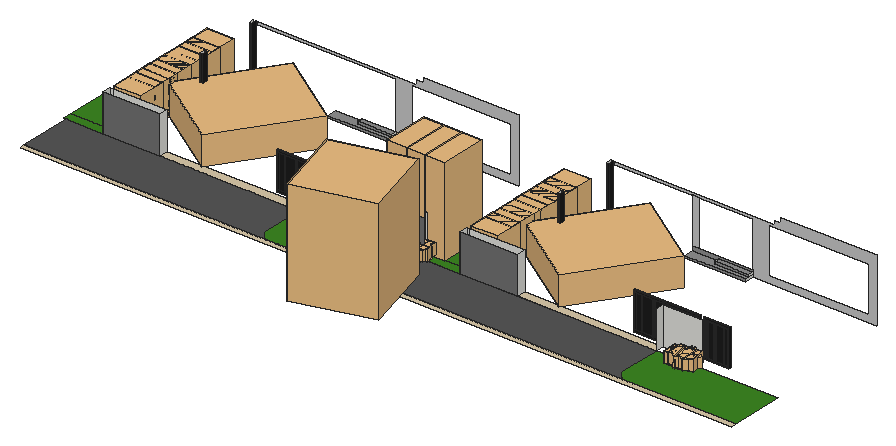
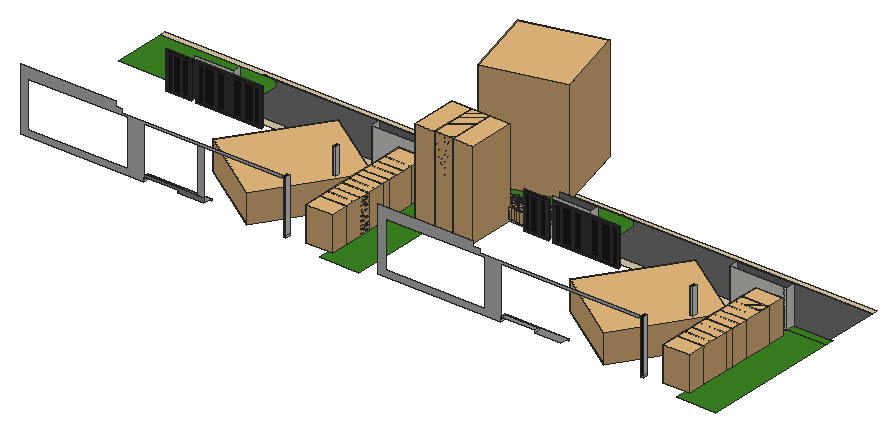
# SketchUp Ruby script. Lengths in inches.
U = 1.inch
M = Sketchup.active_model
def pt(a) = Geom::Point3d.new(a.map { |v| v * U })
def face(e, loops, mat)
  f = e.add_face(loops[0].map { |a| pt(a) })
  loops[1..].each { |l| e.add_face(l.map { |a| pt(a) }).erase! }
  f.material = f.back_material = mat if mat
  f
end
# faces: each face lists its corners as indices into pts; further lists are holes
def faces(e, pts, list, mat = nil) = list.each { |f| face(e, (f[0].is_a?(Array) ? f : [f]).map { |l| l.map { |i| pts[i] } }, mat) }
# xy, xz, yz: faces in a plane at the given z, y or x. An outline is a flat list of corners, or four numbers for a rectangle; further outlines are holes
def ring(l) = l.size == 4 ? [[l[0], l[1]], [l[2], l[1]], [l[2], l[3]], [l[0], l[3]]] : l.each_slice(2).to_a
def flat(e, list, mat, &to3) = list.each { |f| face(e, (f[0].is_a?(Array) ? f : [f]).map { |l| ring(l).map { |u, v| to3.(u, v) } }, mat) }
def xy(e, z, list, mat = nil) = flat(e, list, mat) { |x, y| [x, y, z] }
def xz(e, y, list, mat = nil) = flat(e, list, mat) { |x, z| [x, y, z] }
def yz(e, x, list, mat = nil) = flat(e, list, mat) { |y, z| [x, y, z] }
def lines(e, pts, list) = list.each { |a, b| e.add_line(pt(pts[a]), pt(pts[b])) }
# prism: a flat outline (further loops are holes) pulled along v
def prism(e, loops, v, mat = nil)
  f = face(e, loops, mat); d = Geom::Vector3d.new(v.map { |x| x * U })
  f.pushpull(f.normal.samedirection?(d) ? d.length : -d.length)
end
def box(e, o, s, mat = nil) = prism(e, [[o, [o[0] + s[0], o[1], o[2]], [o[0] + s[0], o[1] + s[1], o[2]], [o[0], o[1] + s[1], o[2]]]], [0, 0, s[2]], mat)
def at(x, y, z, deg = 0) = Geom::Transformation.translation(pt([x, y, z])) * Geom::Transformation.rotation(ORIGIN, Z_AXIS, deg.degrees)
def axes(o, x, y, z) = Geom::Transformation.new([*x, 0, *y, 0, *z, 0, *pt(o).to_a, 1])
def part(name) = M.definitions.add(name)
# library, detail: a bought-in or finely detailed component or shape, given as its bounding box
def library(name, o, s) = part(name).tap { |d| box(d.entities, o, s) }
def detail(e, o, s) = box(e.add_group.entities, o, s)
def put(e, d, t, mat = nil) = e.add_instance(d, t).tap { |i| i.material = mat if mat }
def group(e, t, mat = nil) = e.add_group.tap { |g| g.transformation = t; g.material = mat if mat }.entities
root = M.entities
M.materials.add("[Color M02]").color = [198, 198, 198]
M.materials.add("[Color M04]").color = [60, 133, 34]
M.materials.add("[Color M04]1").color = [142, 142, 142]
M.materials.add("[Color M05]1").color = [114, 114, 114]
M.materials.add("[Color M08]").color = [30, 30, 30]
M.materials.add("[Color_F16]").color = [51, 102, 0]
M.materials.add("[Field Square Tile]").color = [217, 201, 169]
M.materials.add("[Slate Light Tile]").color = [86, 86, 86]
c1 = library("plant (1)",[-35.72,-28.42,0],[66.31,67.39,84.38])
c2 = library("002+Bmw+M4+++mat3.4+2017",[-252.8,19.48,9.01],[196.94,171.32,55.15])
c3 = part("Group\#102")
g1 = group(c3.entities,at(0,0,0))
prism(g1,[[[0,3,72],[70.5,3,72],[70.5,3,0],[0,3,0]],[[67.5,3,3],[67.5,3,69],[3,3,69],[3,3,3]]],[0,-3,0])
c4 = part("Group\#135")
box(c4.entities,[0,0,0],[0.5,1,66])
c5 = part("Group\#148")
box(c5.entities,[0,-1,0],[5.5,1,66])
box(c5.entities,[50.84,-1,0],[13.66,1,66])
box(c5.entities,[28.06,-1,0],[22.28,1,66])
box(c5.entities,[24.66,-1,0],[2.9,1,66])
box(c5.entities,[6,-1,0],[18.16,1,66])
c6 = part("Component\#23")
g2 = group(c6.entities,at(70.5,0,0),"[Color M08]")
put(g2,c3,axes([70.5,0,0],[-1,0,0],[0,1,0],[0,0,1]))
g3 = group(g2,at(3,2,3))
g4 = group(g3,at(0,-1,0))
box(g4,[0,0,0],[5.5,1,66])
box(g4,[50.84,0,0],[13.66,1,66])
box(g4,[28.06,0,0],[22.28,1,66])
box(g4,[24.66,0,0],[2.9,1,66])
box(g4,[6,0,0],[18.16,1,66])
put(g3,c4,axes([50.34,0,0],[1,0,0],[0,-1,0],[0,0,1]))
put(g3,c4,axes([24.16,0,0],[1,0,0],[0,-1,0],[0,0,1]))
put(g3,c4,axes([27.56,0,0],[1,0,0],[0,-1,0],[0,0,1]))
put(g3,c4,axes([5.5,0,0],[1,0,0],[0,-1,0],[0,0,1]))
g5 = group(c6.entities,at(70.5,0,0),"[Color M08]")
put(g5,c3,at(-70.5,0,0))
g6 = group(g5,at(-3,2,3,-180))
put(g6,c5,at(0,1,0))
put(g6,c4,at(50.34,0,0))
put(g6,c4,at(24.16,0,0))
put(g6,c4,at(27.56,0,0))
put(g6,c4,at(5.5,0,0))
g7 = group(c6.entities,at(150,0,0),"[Color M08]")
put(g7,c3,axes([54,0,0],[-0.76596,0,0],[0,1,0],[0,0,1]))
g8 = group(g7,at(2.3,2,3))
put(g8,c5,axes([0,-1,0],[0.76596,0,0],[0,-1,0],[0,0,1]))
put(g8,c4,axes([38.55,0,0],[0.76596,0,0],[0,-1,0],[0,0,1]))
put(g8,c4,axes([18.5,0,0],[0.76596,0,0],[0,-1,0],[0,0,1]))
put(g8,c4,axes([21.11,0,0],[0.76596,0,0],[0,-1,0],[0,0,1]))
put(g8,c4,axes([4.22,0,0],[0.76596,0,0],[0,-1,0],[0,0,1]))
c7 = library("Obj_000004",[-25.54,-25.36,-14.31],[50.67,50.64,41.42])
c8 = library("Obj_000003",[-31,-31.06,-7.89],[62,62.12,39.58])
c9 = library("Potted plant",[-29.7,0,-10.87],[31.67,38.52,72.45])
c10 = library("Palm tree",[-4.09,-4.52,0],[193.52,193.51,258.93])
c11 = part("Palm+Tree")
put(c11.entities,c10,at(25.51,-21.81,0,15))
xy(root,-19.75,[[690.23,10.6,695.34,11.14,700.32,12.39,677.89,12.39,680.03,11.68,685.09,10.78],[1576.69,10.6,1581.8,11.14,1586.78,12.39,1564.35,12.39,1566.5,11.68,1571.56,10.78],[749.87,12.09,755.08,12.39,743.38,12.39,744.65,12.24],[165.7,143.39,173.14,164.82],[173.14,143.39,308.39,164.82],
  [1052.17,143.39,1059.6,164.82],[1059.6,143.39,1194.85,164.82],[264.14,322.71,270.875,334.4375],[1150.61,322.71,1157.34,334.4375],[264.14,475.3125,270.875,487.3125],
  [1150.61,475.3125,1157.34,487.3125]])
xy(root,-19.75,[[677.89,12.39,955.37,12.39,955.37,143.39,653.09,143.39,653.09,39.89,654.46,34.93,656.52,30.23,659.21,25.85,662.49,21.9,666.29,18.4375,670.54,15.55,675.15,13.28],[955.37,12.39,962.46,143.39],[1564.35,12.39,1841.83,12.39,1841.83,143.39,1539.55,143.39,1539.55,39.89,1540.93,34.93,1542.98,30.23,1545.68,25.85,1548.96,21.9,1552.76,18.4375,1557.01,15.55,1561.62,13.28],[68.91,143.39,165.7,164.82],[955.37,143.39,1052.17,164.82],
  [68.91,164.82,165.7,505.3125],[955.37,164.82,1052.17,505.3125]],"[Color M04]")
xy(root,-19.75,[[308.39,143.39,653.09,164.82],[1194.85,143.39,1539.55,164.82]],"[Field Square Tile]")
xy(root,-19.75,[[75.99,12.39,677.89,12.39,675.15,13.28,670.54,15.55,666.29,18.4375,662.49,21.9,659.21,25.85,656.52,30.23,654.46,34.93,653.09,39.89,653.09,143.39,75.99,143.39],[962.46,12.39,1564.35,12.39,1561.62,13.28,1557.01,15.55,1552.76,18.4375,1548.96,21.9,1545.68,25.85,1542.98,30.23,1540.93,34.93,1539.55,39.89,1539.55,143.39,962.46,143.39]],"[Slate Light Tile]")
xy(root,-19.3125,[[75.99,0,955.37,12.39],[955.37,0,962.46,12.39],[962.46,0,1841.83,12.39]],"[Field Square Tile]")
xy(root,-14.01,[[468.02,464.0625,618.43,464.0625,618.43,474.5625,534.06,474.5625,534.06,487.3125,468.02,487.3125],[1354.48,464.0625,1504.89,464.0625,1504.89,474.5625,1420.52,474.5625,1420.52,487.3125,1354.48,487.3125]],"[Color M04]1")
xy(root,-8.01,[[534.06,474.5625,618.43,487.3125],[1420.52,474.5625,1504.89,487.3125]],"[Color M04]1")
xz(root,12.39,[[75.99,-19.75,700.32,-19.3125],[700.32,-19.75,955.37,-19.3125],[955.37,-19.75,962.46,-19.3125],[962.46,-19.75,1586.78,-19.3125]])
xz(root,143.39,[[165.7,-19.75,308.39,73],[653.09,-19.75,962.46,-19.75,962.46,73,901.18,73,901.18,9.9375,747.55,9.9375,747.55,73,653.09,73],[1052.17,-19.75,1194.85,73]],"[Color M05]1")
xz(root,164.82,[[165.7,-19.75,173.14,73],[173.14,-19.75,173.14,73,308.39,73,308.39,-19.75,274.58,-19.75,274.58,-15.625,260.77,-15.625,260.77,-19.75],[260.77,-19.75,274.58,-15.625],[653.09,-19.75,747.55,73],[747.55,-19.75,901.18,9.9375],
  [901.18,-19.75,951.9375,73],[1052.17,-19.75,1059.6,73],[1059.6,-19.75,1059.6,73,1194.85,73,1194.85,-19.75,1161.04,-19.75,1161.04,-15.625,1147.23,-15.625,1147.23,-19.75],[1147.23,-19.75,1161.04,-15.625],[1539.55,-19.75,1634.02,73]])
xz(root,322.71,[[264.14,-19.75,270.875,-15.625],[1150.61,-19.75,1157.34,-15.625]])
xz(root,322.71,[[264.14,-15.625,270.875,115.91],[1150.61,-15.625,1157.34,115.91]],"[Color M08]")
xz(root,334.4375,[[264.14,-19.75,270.875,-15.625],[1150.61,-19.75,1157.34,-15.625],[264.14,-15.625,270.875,115.91],[1150.61,-15.625,1157.34,115.91]])
xz(root,464.0625,[[468.02,-19.75,618.43,-14.01],[1354.48,-19.75,1504.89,-14.01]],"[Color M04]1")
xz(root,474.5625,[[534.06,-14.01,618.43,-8.01],[1420.52,-14.01,1504.89,-8.01]],"[Color M04]1")
xz(root,475.3125,[[264.14,-19.75,270.875,-15.625],[1150.61,-19.75,1157.34,-15.625]])
xz(root,475.3125,[[264.14,-15.625,270.875,115.91],[1150.61,-15.625,1157.34,115.91]],"[Color M08]")
xz(root,487.3125,[[264.14,-19.75,270.875,-15.625],[1150.61,-19.75,1157.34,-15.625],[1150.61,-15.625,1157.34,110.1875]])
xz(root,487.3125,[[[618.43,-19.75,923.77,-19.75,923.77,136.125,686.84,136.125,686.84,125.0625,671.22,125.0625,671.22,123.92,670.9,123.92,670.9,117.06,671.22,117.06,671.22,115.91,275.36,115.91,275.36,110.1875,618.43,110.1875],[658.22,-3.75,903.98,110.1875]],[[1504.89,-19.75,1810.23,-19.75,1810.23,136.125,1573.31,136.125,1573.31,125.0625,1557.68,125.0625,1557.68,123.92,1557.37,123.92,1557.37,117.06,1557.68,117.06,1557.68,115.91,1161.82,115.91,1161.82,110.1875,1504.89,110.1875],[1544.68,-3.75,1790.45,110.1875]],[1354.48,-2.375,1369.77,110.1875]],"[Color M02]")
xz(root,487.3125,[[1354.48,-14.01,1420.52,-14.01,1420.52,-8.01,1504.89,-8.01,1504.89,-2.375,1354.48,-2.375]],"[Color M04]1")
yz(root,165.7,[[143.39,-19.75,164.82,73]])
yz(root,264.14,[[322.71,-19.75,334.4375,-15.625],[475.3125,-19.75,487.3125,-15.625],[322.71,-15.625,334.4375,115.66],[475.3125,-15.625,487.3125,115.66]])
yz(root,270.875,[[322.71,-19.75,334.4375,-15.625],[475.3125,-19.75,487.3125,-15.625]])
yz(root,270.875,[[322.71,-15.625,334.4375,115.91],[475.3125,-15.625,487.3125,115.91]],"[Color M08]")
yz(root,308.39,[[143.39,-19.75,164.82,73]])
yz(root,534.06,[[474.5625,-14.01,487.3125,-8.01]])
yz(root,618.43,[[464.0625,-19.75,487.3125,-14.01],[474.5625,-14.01,487.3125,-8.01]])
yz(root,653.09,[[143.39,-19.75,164.82,73]])
yz(root,1052.17,[[143.39,-19.75,164.82,73]])
yz(root,1150.61,[[322.71,-19.75,334.4375,-15.625],[475.3125,-19.75,487.3125,-15.625],[322.71,-15.625,334.4375,115.66],[475.3125,-15.625,487.3125,115.66]])
yz(root,1157.34,[[322.71,-19.75,334.4375,-15.625],[475.3125,-19.75,487.3125,-15.625]])
yz(root,1157.34,[[322.71,-15.625,334.4375,115.91],[475.3125,-15.625,487.3125,115.91]],"[Color M08]")
yz(root,1194.85,[[143.39,-19.75,164.82,73]])
yz(root,1420.52,[[474.5625,-14.01,487.3125,-8.01]])
yz(root,1504.89,[[464.0625,-19.75,487.3125,-14.01],[474.5625,-14.01,487.3125,-8.01]])
yz(root,1539.55,[[143.39,-19.75,164.82,73]])
p = [[68.91,0,-19.3125],[75.99,0,-19.3125],[75.99,12.39,-19.75],[68.91,12.39,-19.75],[75.99,12.39,-19.3125],[68.91,12.39,-19.3125]]
lines(root,p,[[0,1],[2,3],[4,5]])
put(root,c1,at(193.25,216.8,-19.75))
put(root,c1,at(193.25,261.11,-19.75))
put(root,c1,at(193.25,305.42,-19.75))
put(root,c1,at(193.25,349.73,-19.75))
put(root,c1,at(193.25,394.05,-19.75))
put(root,c1,at(193.25,438.36,-19.75))
put(root,c2,axes([601.1875,415.92,-31.37],[0.71831,1.07151,0],[-1.07151,0.71831,0],[0,0,1.29]))
put(root,c6,axes([571.94,175.05,-19.75],[1.16,0,0],[0,1.16,0],[0,0,1.28819]))
put(root,c7,axes([711.89,130.26,-8.96],[0.64,0,0],[0,0.64,0],[0,0,0.64]))
put(root,c7,axes([727.76,130.26,-8.96],[0.64,0,0],[0,0.64,0],[0,0,0.64]))
put(root,c8,axes([727.76,130.26,-8.96],[0.64,0,0],[0,0.64,0],[0,0,0.64]),"[Color_F16]")
put(root,c7,axes([728.17,130.18,-8.96],[0.45255,0.45255,-0.00035],[-0.45255,0.45255,0.00015],[0.00035,0.00015,0.64]))
put(root,c8,axes([728.17,130.18,-8.96],[0.45255,0.45255,-0.00035],[-0.45255,0.45255,0.00015],[0.00035,0.00015,0.64]),"[Color_F16]")
put(root,c8,axes([744,131.13,-8.96],[-0.54627,0.33345,-0.00035],[-0.33345,-0.54627,0.00015],[-0.00023,0.00031,0.64]),"[Color_F16]")
put(root,c8,axes([744.02,130.71,-8.96],[-0.15049,0.62206,0],[-0.62206,-0.15049,0],[0,0,0.64]),"[Color_F16]")
put(root,c7,axes([744.02,130.71,-8.96],[-0.15049,0.62206,0],[-0.62206,-0.15049,0],[0,0,0.64]))
put(root,c7,axes([744,131.13,-8.96],[-0.54627,0.33345,-0.00035],[-0.33345,-0.54627,0.00015],[-0.00023,0.00031,0.64]))
put(root,c7,axes([759.51,130.26,-8.96],[0.64,0,0],[0,0.64,0],[0,0,0.64]))
put(root,c8,axes([759.51,130.26,-8.96],[0.64,0,0],[0,0.64,0],[0,0,0.64]),"[Color_F16]")
put(root,c7,axes([759.92,130.18,-8.96],[0.45255,0.45255,-0.00035],[-0.45255,0.45255,0.00015],[0.00035,0.00015,0.64]))
put(root,c8,axes([759.92,130.18,-8.96],[0.45255,0.45255,-0.00035],[-0.45255,0.45255,0.00015],[0.00035,0.00015,0.64]),"[Color_F16]")
put(root,c7,axes([775.38,130.26,-8.96],[0.64,0,0],[0,0.64,0],[0,0,0.64]))
put(root,c8,axes([775.38,130.26,-8.96],[0.64,0,0],[0,0.64,0],[0,0,0.64]),"[Color_F16]")
put(root,c7,axes([775.79,130.18,-8.96],[0.45255,0.45255,-0.00035],[-0.45255,0.45255,0.00015],[0.00035,0.00015,0.64]))
put(root,c8,axes([775.79,130.18,-8.96],[0.45255,0.45255,-0.00035],[-0.45255,0.45255,0.00015],[0.00035,0.00015,0.64]),"[Color_F16]")
put(root,c7,axes([790.97,130.52,-8.96],[0.28256,0.57425,0],[-0.57425,0.28256,0],[0,0,0.64]))
put(root,c8,axes([791.22,130.86,-8.96],[-0.20625,0.60586,-0.00035],[-0.60586,-0.20625,0.00015],[0.00002,0.00038,0.64]),"[Color_F16]")
put(root,c8,axes([791.26,130.26,-8.96],[0.64,0,0],[0,0.64,0],[0,0,0.64]),"[Color_F16]")
put(root,c7,axes([791.22,130.86,-8.96],[-0.20625,0.60586,-0.00035],[-0.60586,-0.20625,0.00015],[0.00002,0.00038,0.64]))
put(root,c7,axes([805.73,144.21,-8.16],[0.64,0,0],[0,0.64,0],[0,0,0.64]))
put(root,c7,axes([821.6,144.21,-8.16],[0.64,0,0],[0,0.64,0],[0,0,0.64]))
put(root,c8,axes([821.6,144.21,-8.16],[0.64,0,0],[0,0.64,0],[0,0,0.64]),"[Color_F16]")
put(root,c7,axes([822.01,144.13,-8.16],[0.45255,0.45255,-0.00035],[-0.45255,0.45255,0.00015],[0.00035,0.00015,0.64]))
put(root,c8,axes([822.01,144.13,-8.16],[0.45255,0.45255,-0.00035],[-0.45255,0.45255,0.00015],[0.00035,0.00015,0.64]),"[Color_F16]")
put(root,c8,axes([837.84,145.08,-8.16],[-0.54627,0.33345,-0.00035],[-0.33345,-0.54627,0.00015],[-0.00023,0.00031,0.64]),"[Color_F16]")
put(root,c8,axes([837.86,144.66,-8.16],[-0.15049,0.62206,0],[-0.62206,-0.15049,0],[0,0,0.64]),"[Color_F16]")
put(root,c7,axes([837.86,144.66,-8.16],[-0.15049,0.62206,0],[-0.62206,-0.15049,0],[0,0,0.64]))
put(root,c7,axes([837.84,145.08,-8.16],[-0.54627,0.33345,-0.00035],[-0.33345,-0.54627,0.00015],[-0.00023,0.00031,0.64]))
put(root,c7,axes([853.35,144.21,-8.16],[0.64,0,0],[0,0.64,0],[0,0,0.64]))
put(root,c8,axes([853.35,144.21,-8.16],[0.64,0,0],[0,0.64,0],[0,0,0.64]),"[Color_F16]")
put(root,c7,axes([853.76,144.13,-8.16],[0.45255,0.45255,-0.00035],[-0.45255,0.45255,0.00015],[0.00035,0.00015,0.64]))
put(root,c8,axes([853.76,144.13,-8.16],[0.45255,0.45255,-0.00035],[-0.45255,0.45255,0.00015],[0.00035,0.00015,0.64]),"[Color_F16]")
put(root,c7,axes([869.22,144.21,-8.16],[0.64,0,0],[0,0.64,0],[0,0,0.64]))
put(root,c8,axes([869.22,144.21,-8.16],[0.64,0,0],[0,0.64,0],[0,0,0.64]),"[Color_F16]")
put(root,c7,axes([869.63,144.13,-8.16],[0.45255,0.45255,-0.00035],[-0.45255,0.45255,0.00015],[0.00035,0.00015,0.64]))
put(root,c8,axes([869.63,144.13,-8.16],[0.45255,0.45255,-0.00035],[-0.45255,0.45255,0.00015],[0.00035,0.00015,0.64]),"[Color_F16]")
put(root,c7,axes([876.1,144.21,-8.16],[0.64,0,0],[0,0.64,0],[0,0,0.64]))
put(root,c7,axes([884.81,144.47,-8.16],[0.28256,0.57425,0],[-0.57425,0.28256,0],[0,0,0.64]))
put(root,c8,axes([885.06,144.81,-8.16],[-0.20625,0.60586,-0.00035],[-0.60586,-0.20625,0.00015],[0.00002,0.00038,0.64]),"[Color_F16]")
put(root,c8,axes([885.1,144.21,-8.16],[0.64,0,0],[0,0.64,0],[0,0,0.64]),"[Color_F16]")
put(root,c7,axes([885.06,144.81,-8.16],[-0.20625,0.60586,-0.00035],[-0.60586,-0.20625,0.00015],[0.00002,0.00038,0.64]))
put(root,c7,axes([891.97,144.21,-8.16],[0.64,0,0],[0,0.64,0],[0,0,0.64]))
put(root,c8,axes([891.97,144.21,-8.16],[0.64,0,0],[0,0.64,0],[0,0,0.64]),"[Color_F16]")
put(root,c7,axes([892.38,144.13,-8.16],[0.45255,0.45255,-0.00035],[-0.45255,0.45255,0.00015],[0.00035,0.00015,0.64]))
put(root,c8,axes([892.38,144.13,-8.16],[0.45255,0.45255,-0.00035],[-0.45255,0.45255,0.00015],[0.00035,0.00015,0.64]),"[Color_F16]")
put(root,c9,axes([942.04,164.82,12.86],[3,0,0],[0,3,0],[0,0,3]))
put(root,c8,axes([908.21,145.08,-8.16],[-0.54627,0.33345,-0.00035],[-0.33345,-0.54627,0.00015],[-0.00023,0.00031,0.64]),"[Color_F16]")
put(root,c8,axes([908.23,144.66,-8.16],[-0.15049,0.62206,0],[-0.62206,-0.15049,0],[0,0,0.64]),"[Color_F16]")
put(root,c7,axes([908.23,144.66,-8.16],[-0.15049,0.62206,0],[-0.62206,-0.15049,0],[0,0,0.64]))
put(root,c7,axes([908.21,145.08,-8.16],[-0.54627,0.33345,-0.00035],[-0.33345,-0.54627,0.00015],[-0.00023,0.00031,0.64]))
put(root,c7,axes([923.72,144.21,-8.16],[0.64,0,0],[0,0.64,0],[0,0,0.64]))
put(root,c8,axes([923.72,144.21,-8.16],[0.64,0,0],[0,0.64,0],[0,0,0.64]),"[Color_F16]")
put(root,c7,axes([924.13,144.13,-8.16],[0.45255,0.45255,-0.00035],[-0.45255,0.45255,0.00015],[0.00035,0.00015,0.64]))
put(root,c8,axes([924.13,144.13,-8.16],[0.45255,0.45255,-0.00035],[-0.45255,0.45255,0.00015],[0.00035,0.00015,0.64]),"[Color_F16]")
put(root,c11,at(837.38,-125.125,-17.22))
put(root,c7,axes([939.6,144.21,-8.16],[0.64,0,0],[0,0.64,0],[0,0,0.64]))
put(root,c8,axes([939.6,144.21,-8.16],[0.64,0,0],[0,0.64,0],[0,0,0.64]),"[Color_F16]")
put(root,c7,axes([940.01,144.13,-8.16],[0.45255,0.45255,-0.00035],[-0.45255,0.45255,0.00015],[0.00035,0.00015,0.64]))
put(root,c8,axes([940.01,144.13,-8.16],[0.45255,0.45255,-0.00035],[-0.45255,0.45255,0.00015],[0.00035,0.00015,0.64]),"[Color_F16]")
put(root,c9,axes([991.91,164.82,12.86],[3,0,0],[0,3,0],[0,0,3]))
put(root,c7,axes([955.18,144.47,-8.16],[0.28256,0.57425,0],[-0.57425,0.28256,0],[0,0,0.64]))
put(root,c8,axes([955.43,144.81,-8.16],[-0.20625,0.60586,-0.00035],[-0.60586,-0.20625,0.00015],[0.00002,0.00038,0.64]),"[Color_F16]")
put(root,c8,axes([955.47,144.21,-8.16],[0.64,0,0],[0,0.64,0],[0,0,0.64]),"[Color_F16]")
put(root,c7,axes([955.43,144.81,-8.16],[-0.20625,0.60586,-0.00035],[-0.60586,-0.20625,0.00015],[0.00002,0.00038,0.64]))
put(root,c1,at(1079.72,216.8,-19.75))
put(root,c1,at(1079.72,261.11,-19.75))
put(root,c1,at(1079.72,305.42,-19.75))
put(root,c1,at(1079.72,349.73,-19.75))
put(root,c1,at(1079.72,394.05,-19.75))
put(root,c1,at(1079.72,438.36,-19.75))
put(root,c2,axes([1487.65,415.92,-31.37],[0.71831,1.07151,0],[-1.07151,0.71831,0],[0,0,1.29]))
put(root,c6,axes([1458.41,175.05,-19.75],[1.16,0,0],[0,1.16,0],[0,0,1.28819]))
put(root,c7,axes([1598.35,130.26,-8.96],[0.64,0,0],[0,0.64,0],[0,0,0.64]))
put(root,c7,axes([1614.23,130.26,-8.96],[0.64,0,0],[0,0.64,0],[0,0,0.64]))
put(root,c8,axes([1614.23,130.26,-8.96],[0.64,0,0],[0,0.64,0],[0,0,0.64]),"[Color_F16]")
put(root,c7,axes([1614.64,130.18,-8.96],[0.45255,0.45255,-0.00035],[-0.45255,0.45255,0.00015],[0.00035,0.00015,0.64]))
put(root,c8,axes([1614.64,130.18,-8.96],[0.45255,0.45255,-0.00035],[-0.45255,0.45255,0.00015],[0.00035,0.00015,0.64]),"[Color_F16]")
put(root,c8,axes([1630.46,131.13,-8.96],[-0.54627,0.33345,-0.00035],[-0.33345,-0.54627,0.00015],[-0.00023,0.00031,0.64]),"[Color_F16]")
put(root,c8,axes([1630.48,130.71,-8.96],[-0.15049,0.62206,0],[-0.62206,-0.15049,0],[0,0,0.64]),"[Color_F16]")
put(root,c7,axes([1630.48,130.71,-8.96],[-0.15049,0.62206,0],[-0.62206,-0.15049,0],[0,0,0.64]))
